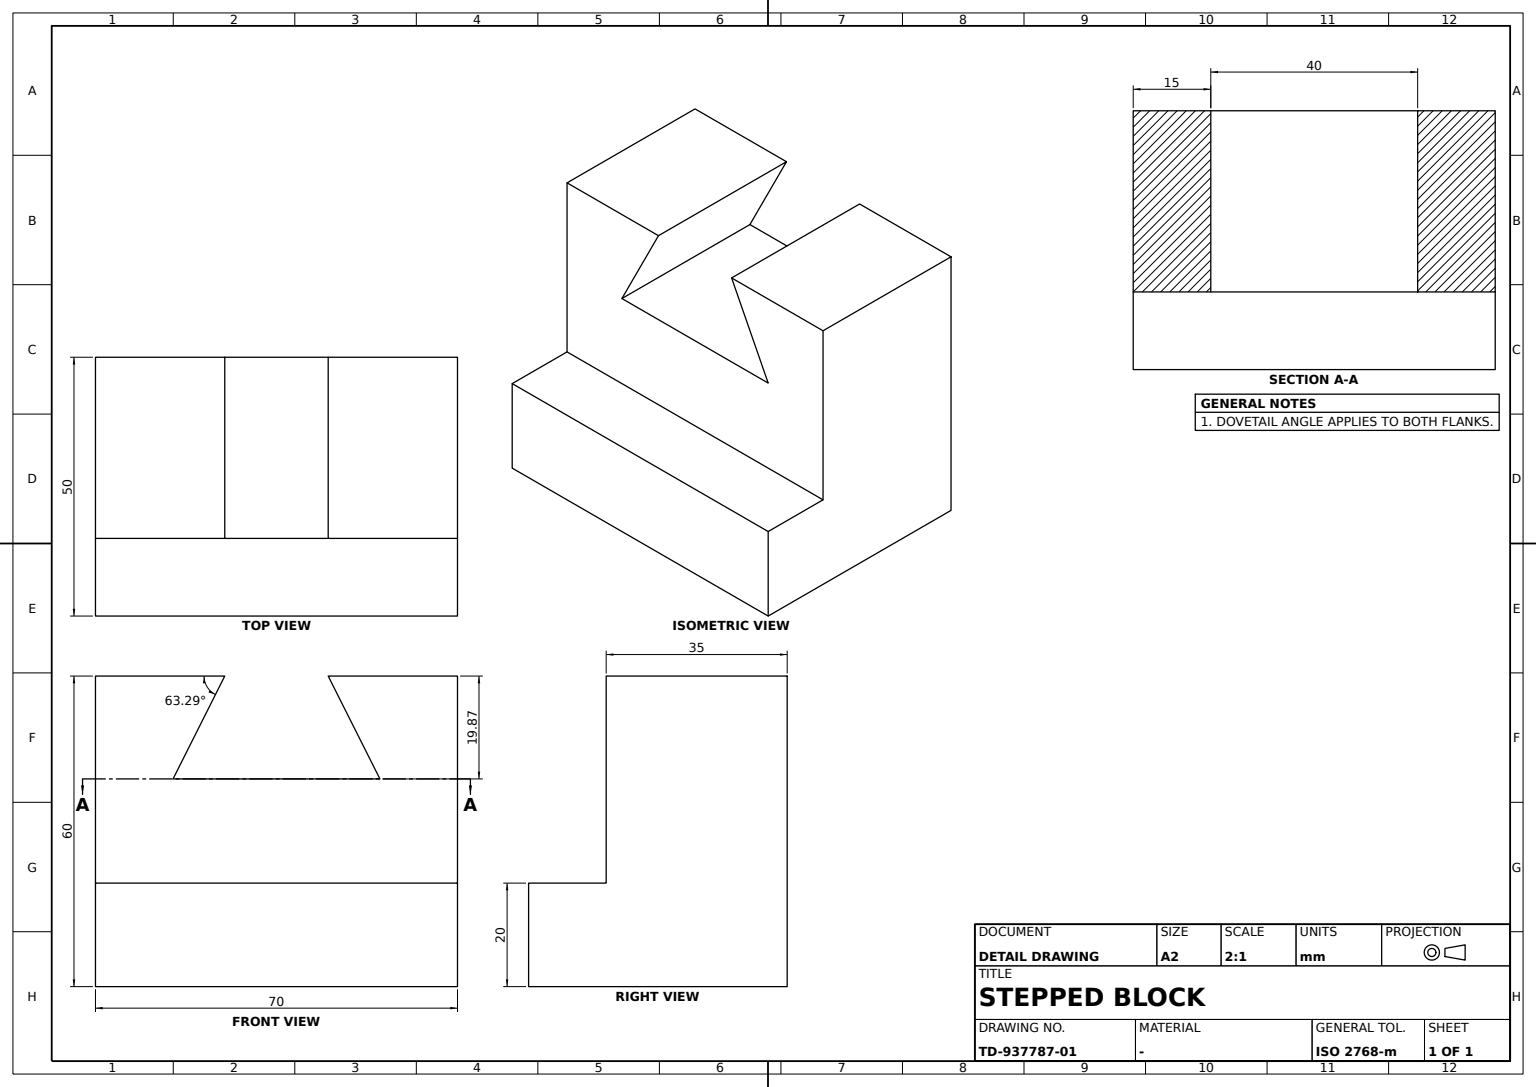
ISO-10303-21;
HEADER;
FILE_DESCRIPTION((''),'2;1');
FILE_NAME('','',(''),(''),'','','');
FILE_SCHEMA(('AUTOMOTIVE_DESIGN'));
ENDSEC;
DATA;
#1=APPLICATION_CONTEXT('');
#2=PRODUCT_CONTEXT('',#1,'mechanical');
#3=PRODUCT('','','',(#2));
#4=PRODUCT_DEFINITION_FORMATION('','',#3);
#5=PRODUCT_DEFINITION_CONTEXT('',#1,'design');
#6=PRODUCT_DEFINITION('','',#4,#5);
#7=PRODUCT_DEFINITION_SHAPE('','',#6);
#8=(LENGTH_UNIT()NAMED_UNIT(*)SI_UNIT(.MILLI.,.METRE.));
#9=(NAMED_UNIT(*)PLANE_ANGLE_UNIT()SI_UNIT($,.RADIAN.));
#10=(NAMED_UNIT(*)SI_UNIT($,.STERADIAN.)SOLID_ANGLE_UNIT());
#11=UNCERTAINTY_MEASURE_WITH_UNIT(LENGTH_MEASURE(0.005),#8,'distance_accuracy_value','');
#12=(GEOMETRIC_REPRESENTATION_CONTEXT(3)GLOBAL_UNCERTAINTY_ASSIGNED_CONTEXT((#11))GLOBAL_UNIT_ASSIGNED_CONTEXT((#8,#9,#10))REPRESENTATION_CONTEXT('',''));
#13=CARTESIAN_POINT('',(35.,0.,60.));
#14=VERTEX_POINT('',#13);
#15=CARTESIAN_POINT('',(35.,0.,0.));
#16=VERTEX_POINT('',#15);
#17=DIRECTION('',(0.,0.,-1.));
#18=VECTOR('',#17,1000.);
#19=LINE('',#15,#18);
#20=EDGE_CURVE('',#14,#16,#19,.T.);
#21=ORIENTED_EDGE('',*,*,#20,.T.);
#22=CARTESIAN_POINT('',(35.,50.,0.));
#23=VERTEX_POINT('',#22);
#24=DIRECTION('',(0.,1.,0.));
#25=VECTOR('',#24,1000.);
#26=LINE('',#15,#25);
#27=EDGE_CURVE('',#16,#23,#26,.T.);
#28=ORIENTED_EDGE('',*,*,#27,.T.);
#29=CARTESIAN_POINT('',(35.,50.,20.));
#30=VERTEX_POINT('',#29);
#31=DIRECTION('',(0.,0.,1.));
#32=VECTOR('',#31,1000.);
#33=LINE('',#22,#32);
#34=EDGE_CURVE('',#23,#30,#33,.T.);
#35=ORIENTED_EDGE('',*,*,#34,.T.);
#36=CARTESIAN_POINT('',(35.,35.,20.));
#37=VERTEX_POINT('',#36);
#38=CARTESIAN_POINT('',(35.,0.,20.));
#39=DIRECTION('',(0.,-1.,0.));
#40=VECTOR('',#39,1000.);
#41=LINE('',#38,#40);
#42=EDGE_CURVE('',#30,#37,#41,.T.);
#43=ORIENTED_EDGE('',*,*,#42,.T.);
#44=CARTESIAN_POINT('',(35.,35.,60.));
#45=VERTEX_POINT('',#44);
#46=CARTESIAN_POINT('',(35.,35.,0.));
#47=LINE('',#46,#32);
#48=EDGE_CURVE('',#37,#45,#47,.T.);
#49=ORIENTED_EDGE('',*,*,#48,.T.);
#50=LINE('',#13,#40);
#51=EDGE_CURVE('',#45,#14,#50,.T.);
#52=ORIENTED_EDGE('',*,*,#51,.T.);
#53=EDGE_LOOP('',(#21,#28,#35,#43,#49,#52));
#54=FACE_BOUND('',#53,.T.);
#55=DIRECTION('',(1.,0.,0.));
#56=AXIS2_PLACEMENT_3D('',#15,#55,#24);
#57=PLANE('',#56);
#58=ADVANCED_FACE('',(#54),#57,.T.);
#59=CARTESIAN_POINT('',(20.,35.,40.127518));
#60=VERTEX_POINT('',#59);
#61=CARTESIAN_POINT('',(20.,0.,40.127518));
#62=VERTEX_POINT('',#61);
#63=LINE('',#59,#40);
#64=EDGE_CURVE('',#60,#62,#63,.T.);
#65=ORIENTED_EDGE('',*,*,#64,.T.);
#66=CARTESIAN_POINT('',(10.,0.,60.));
#67=VERTEX_POINT('',#66);
#68=DIRECTION('',(0.449504919,0.,-0.893277856));
#69=VECTOR('',#68,1000.);
#70=LINE('',#61,#69);
#71=EDGE_CURVE('',#67,#62,#70,.T.);
#72=ORIENTED_EDGE('',*,*,#71,.F.);
#73=CARTESIAN_POINT('',(10.,35.,60.));
#74=VERTEX_POINT('',#73);
#75=LINE('',#73,#40);
#76=EDGE_CURVE('',#74,#67,#75,.T.);
#77=ORIENTED_EDGE('',*,*,#76,.F.);
#78=DIRECTION('',(-0.449504919,0.,0.893277856));
#79=VECTOR('',#78,1000.);
#80=LINE('',#59,#79);
#81=EDGE_CURVE('',#60,#74,#80,.T.);
#82=ORIENTED_EDGE('',*,*,#81,.F.);
#83=EDGE_LOOP('',(#65,#72,#77,#82));
#84=FACE_BOUND('',#83,.T.);
#85=DIRECTION('',(0.893277856,0.,0.449504919));
#86=AXIS2_PLACEMENT_3D('',#59,#85,#78);
#87=PLANE('',#86);
#88=ADVANCED_FACE('',(#84),#87,.F.);
#89=CARTESIAN_POINT('',(-35.,50.,20.));
#90=VERTEX_POINT('',#89);
#91=CARTESIAN_POINT('',(0.,50.,20.));
#92=VECTOR('',#55,1000.);
#93=LINE('',#91,#92);
#94=EDGE_CURVE('',#90,#30,#93,.T.);
#95=ORIENTED_EDGE('',*,*,#94,.T.);
#96=ORIENTED_EDGE('',*,*,#34,.F.);
#97=CARTESIAN_POINT('',(-35.,50.,0.));
#98=VERTEX_POINT('',#97);
#99=CARTESIAN_POINT('',(0.,50.,0.));
#100=LINE('',#99,#92);
#101=EDGE_CURVE('',#98,#23,#100,.T.);
#102=ORIENTED_EDGE('',*,*,#101,.F.);
#103=LINE('',#97,#32);
#104=EDGE_CURVE('',#98,#90,#103,.T.);
#105=ORIENTED_EDGE('',*,*,#104,.T.);
#106=EDGE_LOOP('',(#95,#96,#102,#105));
#107=FACE_BOUND('',#106,.T.);
#108=AXIS2_PLACEMENT_3D('',#99,#24,#31);
#109=PLANE('',#108);
#110=ADVANCED_FACE('',(#107),#109,.T.);
#111=CARTESIAN_POINT('',(-20.,35.,40.127518));
#112=VERTEX_POINT('',#111);
#113=DIRECTION('',(-1.,0.,0.));
#114=VECTOR('',#113,1000.);
#115=LINE('',#59,#114);
#116=EDGE_CURVE('',#60,#112,#115,.T.);
#117=ORIENTED_EDGE('',*,*,#116,.F.);
#118=ORIENTED_EDGE('',*,*,#81,.T.);
#119=CARTESIAN_POINT('',(0.,35.,60.));
#120=LINE('',#119,#92);
#121=EDGE_CURVE('',#74,#45,#120,.T.);
#122=ORIENTED_EDGE('',*,*,#121,.T.);
#123=ORIENTED_EDGE('',*,*,#48,.F.);
#124=CARTESIAN_POINT('',(-35.,35.,20.));
#125=VERTEX_POINT('',#124);
#126=CARTESIAN_POINT('',(0.,35.,20.));
#127=LINE('',#126,#92);
#128=EDGE_CURVE('',#125,#37,#127,.T.);
#129=ORIENTED_EDGE('',*,*,#128,.F.);
#130=CARTESIAN_POINT('',(-35.,35.,60.));
#131=VERTEX_POINT('',#130);
#132=CARTESIAN_POINT('',(-35.,35.,0.));
#133=LINE('',#132,#32);
#134=EDGE_CURVE('',#125,#131,#133,.T.);
#135=ORIENTED_EDGE('',*,*,#134,.T.);
#136=CARTESIAN_POINT('',(-10.,35.,60.));
#137=VERTEX_POINT('',#136);
#138=EDGE_CURVE('',#131,#137,#120,.T.);
#139=ORIENTED_EDGE('',*,*,#138,.T.);
#140=DIRECTION('',(-0.449504919,0.,-0.893277856));
#141=VECTOR('',#140,1000.);
#142=LINE('',#136,#141);
#143=EDGE_CURVE('',#137,#112,#142,.T.);
#144=ORIENTED_EDGE('',*,*,#143,.T.);
#145=EDGE_LOOP('',(#117,#118,#122,#123,#129,#135,#139,#144));
#146=FACE_BOUND('',#145,.T.);
#147=AXIS2_PLACEMENT_3D('',#126,#24,#31);
#148=PLANE('',#147);
#149=ADVANCED_FACE('',(#146),#148,.T.);
#150=ORIENTED_EDGE('',*,*,#94,.F.);
#151=CARTESIAN_POINT('',(-35.,0.,20.));
#152=LINE('',#151,#40);
#153=EDGE_CURVE('',#90,#125,#152,.T.);
#154=ORIENTED_EDGE('',*,*,#153,.T.);
#155=ORIENTED_EDGE('',*,*,#128,.T.);
#156=ORIENTED_EDGE('',*,*,#42,.F.);
#157=EDGE_LOOP('',(#150,#154,#155,#156));
#158=FACE_BOUND('',#157,.T.);
#159=AXIS2_PLACEMENT_3D('',#91,#31,#39);
#160=PLANE('',#159);
#161=ADVANCED_FACE('',(#158),#160,.T.);
#162=ORIENTED_EDGE('',*,*,#76,.T.);
#163=CARTESIAN_POINT('',(0.,0.,60.));
#164=LINE('',#163,#92);
#165=EDGE_CURVE('',#67,#14,#164,.T.);
#166=ORIENTED_EDGE('',*,*,#165,.T.);
#167=ORIENTED_EDGE('',*,*,#51,.F.);
#168=ORIENTED_EDGE('',*,*,#121,.F.);
#169=EDGE_LOOP('',(#162,#166,#167,#168));
#170=FACE_BOUND('',#169,.T.);
#171=AXIS2_PLACEMENT_3D('',#119,#31,#39);
#172=PLANE('',#171);
#173=ADVANCED_FACE('',(#170),#172,.T.);
#174=ORIENTED_EDGE('',*,*,#138,.F.);
#175=CARTESIAN_POINT('',(-35.,0.,60.));
#176=VERTEX_POINT('',#175);
#177=LINE('',#175,#40);
#178=EDGE_CURVE('',#131,#176,#177,.T.);
#179=ORIENTED_EDGE('',*,*,#178,.T.);
#180=CARTESIAN_POINT('',(-10.,0.,60.));
#181=VERTEX_POINT('',#180);
#182=EDGE_CURVE('',#176,#181,#164,.T.);
#183=ORIENTED_EDGE('',*,*,#182,.T.);
#184=LINE('',#136,#40);
#185=EDGE_CURVE('',#137,#181,#184,.T.);
#186=ORIENTED_EDGE('',*,*,#185,.F.);
#187=EDGE_LOOP('',(#174,#179,#183,#186));
#188=FACE_BOUND('',#187,.T.);
#189=ADVANCED_FACE('',(#188),#172,.T.);
#190=CARTESIAN_POINT('',(-20.,0.,40.127518));
#191=VERTEX_POINT('',#190);
#192=CARTESIAN_POINT('',(0.,0.,40.127518));
#193=LINE('',#192,#114);
#194=EDGE_CURVE('',#62,#191,#193,.T.);
#195=ORIENTED_EDGE('',*,*,#194,.F.);
#196=ORIENTED_EDGE('',*,*,#64,.F.);
#197=ORIENTED_EDGE('',*,*,#116,.T.);
#198=LINE('',#111,#40);
#199=EDGE_CURVE('',#112,#191,#198,.T.);
#200=ORIENTED_EDGE('',*,*,#199,.T.);
#201=EDGE_LOOP('',(#195,#196,#197,#200));
#202=FACE_BOUND('',#201,.T.);
#203=AXIS2_PLACEMENT_3D('',#59,#31,#113);
#204=PLANE('',#203);
#205=ADVANCED_FACE('',(#202),#204,.T.);
#206=CARTESIAN_POINT('',(-35.,0.,0.));
#207=VERTEX_POINT('',#206);
#208=CARTESIAN_POINT('',(0.,0.,0.));
#209=LINE('',#208,#92);
#210=EDGE_CURVE('',#207,#16,#209,.T.);
#211=ORIENTED_EDGE('',*,*,#210,.F.);
#212=LINE('',#206,#25);
#213=EDGE_CURVE('',#207,#98,#212,.T.);
#214=ORIENTED_EDGE('',*,*,#213,.T.);
#215=ORIENTED_EDGE('',*,*,#101,.T.);
#216=ORIENTED_EDGE('',*,*,#27,.F.);
#217=EDGE_LOOP('',(#211,#214,#215,#216));
#218=FACE_BOUND('',#217,.T.);
#219=AXIS2_PLACEMENT_3D('',#208,#17,#24);
#220=PLANE('',#219);
#221=ADVANCED_FACE('',(#218),#220,.T.);
#222=ORIENTED_EDGE('',*,*,#143,.F.);
#223=ORIENTED_EDGE('',*,*,#185,.T.);
#224=CARTESIAN_POINT('',(-7.979453,0.,64.015328));
#225=LINE('',#224,#141);
#226=EDGE_CURVE('',#181,#191,#225,.T.);
#227=ORIENTED_EDGE('',*,*,#226,.T.);
#228=ORIENTED_EDGE('',*,*,#199,.F.);
#229=EDGE_LOOP('',(#222,#223,#227,#228));
#230=FACE_BOUND('',#229,.T.);
#231=DIRECTION('',(-0.893277856,0.,0.449504919));
#232=AXIS2_PLACEMENT_3D('',#136,#231,#140);
#233=PLANE('',#232);
#234=ADVANCED_FACE('',(#230),#233,.F.);
#235=ORIENTED_EDGE('',*,*,#20,.F.);
#236=ORIENTED_EDGE('',*,*,#165,.F.);
#237=ORIENTED_EDGE('',*,*,#71,.T.);
#238=ORIENTED_EDGE('',*,*,#194,.T.);
#239=ORIENTED_EDGE('',*,*,#226,.F.);
#240=ORIENTED_EDGE('',*,*,#182,.F.);
#241=LINE('',#206,#18);
#242=EDGE_CURVE('',#176,#207,#241,.T.);
#243=ORIENTED_EDGE('',*,*,#242,.T.);
#244=ORIENTED_EDGE('',*,*,#210,.T.);
#245=EDGE_LOOP('',(#235,#236,#237,#238,#239,#240,#243,#244));
#246=FACE_BOUND('',#245,.T.);
#247=AXIS2_PLACEMENT_3D('',#163,#39,#17);
#248=PLANE('',#247);
#249=ADVANCED_FACE('',(#246),#248,.T.);
#250=ORIENTED_EDGE('',*,*,#178,.F.);
#251=ORIENTED_EDGE('',*,*,#134,.F.);
#252=ORIENTED_EDGE('',*,*,#153,.F.);
#253=ORIENTED_EDGE('',*,*,#104,.F.);
#254=ORIENTED_EDGE('',*,*,#213,.F.);
#255=ORIENTED_EDGE('',*,*,#242,.F.);
#256=EDGE_LOOP('',(#250,#251,#252,#253,#254,#255));
#257=FACE_BOUND('',#256,.T.);
#258=AXIS2_PLACEMENT_3D('',#206,#55,#24);
#259=PLANE('',#258);
#260=ADVANCED_FACE('',(#257),#259,.F.);
#261=CLOSED_SHELL('',(#58,#88,#110,#149,#161,#173,#189,#205,#221,#234,#249,#260));
#262=MANIFOLD_SOLID_BREP('',#261);
#263=ADVANCED_BREP_SHAPE_REPRESENTATION('',(#262),#12);
#264=SHAPE_DEFINITION_REPRESENTATION(#7,#263);
ENDSEC;
END-ISO-10303-21;
